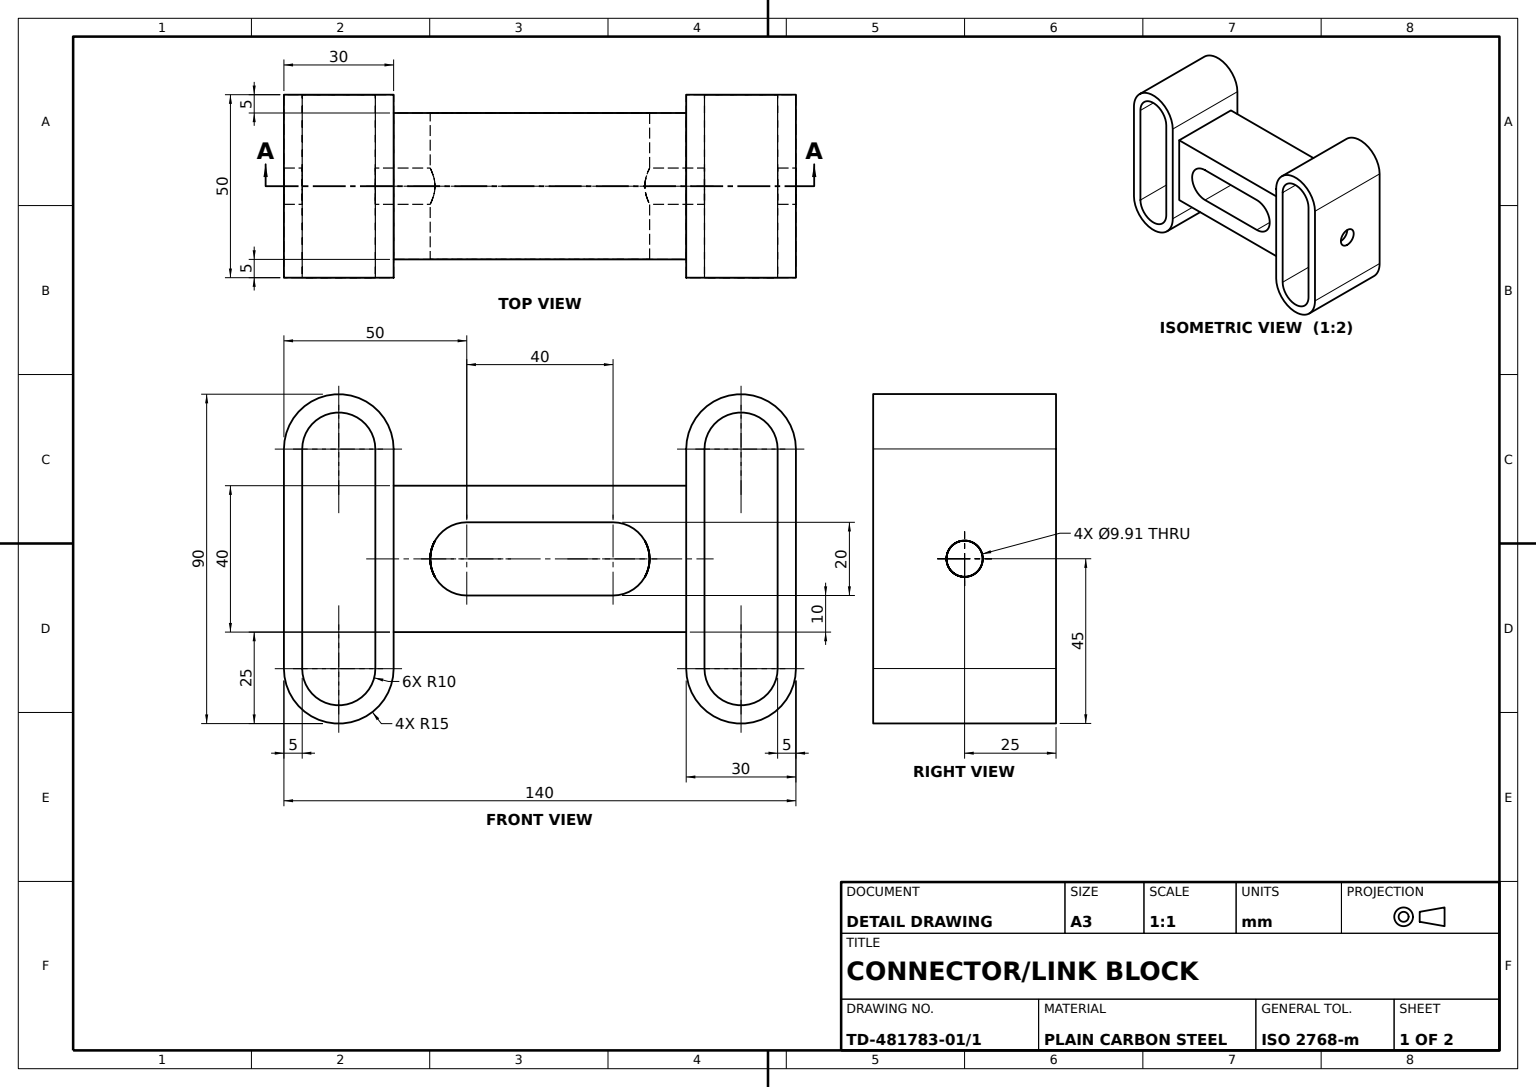
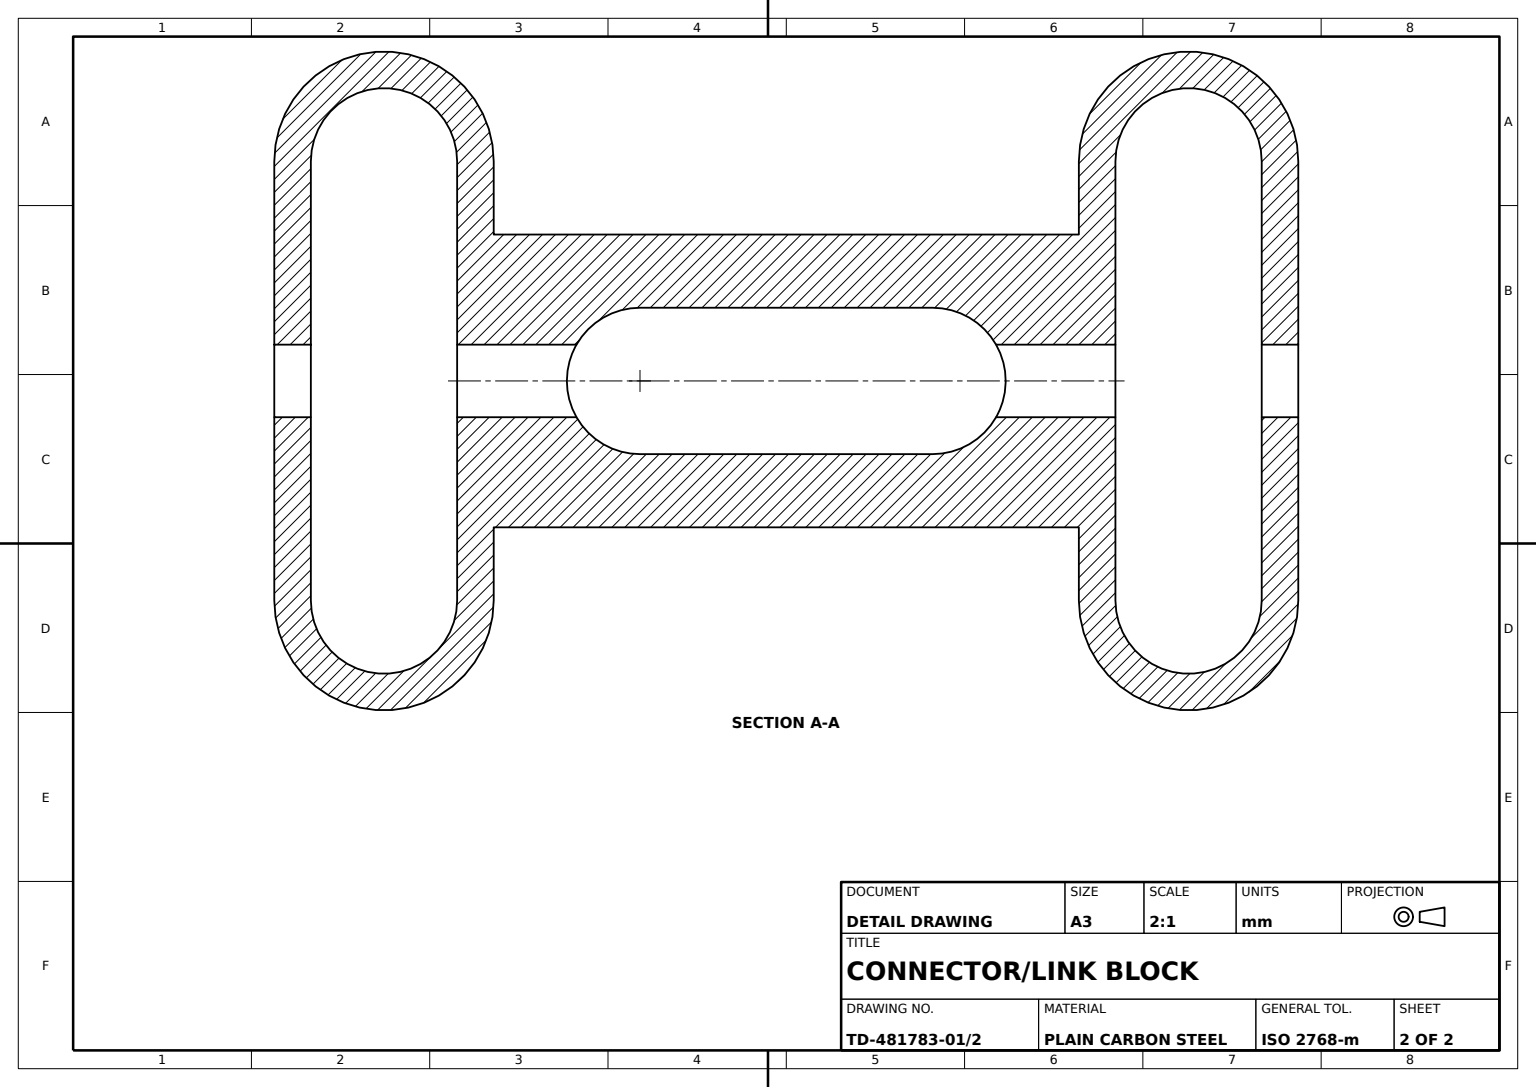
ISO-10303-21;
HEADER;
FILE_DESCRIPTION((''),'2;1');
FILE_NAME('','',(''),(''),'','','');
FILE_SCHEMA(('AUTOMOTIVE_DESIGN'));
ENDSEC;
DATA;
#1=APPLICATION_CONTEXT('');
#2=PRODUCT_CONTEXT('',#1,'mechanical');
#3=PRODUCT('','','',(#2));
#4=PRODUCT_DEFINITION_FORMATION('','',#3);
#5=PRODUCT_DEFINITION_CONTEXT('',#1,'design');
#6=PRODUCT_DEFINITION('','',#4,#5);
#7=PRODUCT_DEFINITION_SHAPE('','',#6);
#8=(LENGTH_UNIT()NAMED_UNIT(*)SI_UNIT(.MILLI.,.METRE.));
#9=(NAMED_UNIT(*)PLANE_ANGLE_UNIT()SI_UNIT($,.RADIAN.));
#10=(NAMED_UNIT(*)SI_UNIT($,.STERADIAN.)SOLID_ANGLE_UNIT());
#11=UNCERTAINTY_MEASURE_WITH_UNIT(LENGTH_MEASURE(1.E-05),#8,'distance_accuracy_value','');
#12=(GEOMETRIC_REPRESENTATION_CONTEXT(3)GLOBAL_UNCERTAINTY_ASSIGNED_CONTEXT((#11))GLOBAL_UNIT_ASSIGNED_CONTEXT((#8,#9,#10))REPRESENTATION_CONTEXT('',''));
#13=CARTESIAN_POINT('',(20.,-5.,20.));
#14=VERTEX_POINT('',#13);
#15=CARTESIAN_POINT('',(20.,15.,20.));
#16=VERTEX_POINT('',#15);
#17=CARTESIAN_POINT('',(20.,5.,20.));
#18=DIRECTION('',(0.,0.,1.));
#19=DIRECTION('',(1.,0.,0.));
#20=AXIS2_PLACEMENT_3D('',#17,#18,#19);
#21=CIRCLE('',#20,10.);
#22=EDGE_CURVE('',#14,#16,#21,.T.);
#23=ORIENTED_EDGE('',*,*,#22,.T.);
#24=CARTESIAN_POINT('',(20.,15.,-20.));
#25=VERTEX_POINT('',#24);
#26=DIRECTION('',(0.,0.,-1.));
#27=VECTOR('',#26,1000.);
#28=LINE('',#15,#27);
#29=EDGE_CURVE('',#16,#25,#28,.T.);
#30=ORIENTED_EDGE('',*,*,#29,.T.);
#31=CARTESIAN_POINT('',(20.,-5.,-20.));
#32=VERTEX_POINT('',#31);
#33=CARTESIAN_POINT('',(20.,5.,-20.));
#34=AXIS2_PLACEMENT_3D('',#33,#18,#19);
#35=CIRCLE('',#34,10.);
#36=EDGE_CURVE('',#32,#25,#35,.T.);
#37=ORIENTED_EDGE('',*,*,#36,.F.);
#38=LINE('',#13,#27);
#39=EDGE_CURVE('',#14,#32,#38,.T.);
#40=ORIENTED_EDGE('',*,*,#39,.F.);
#41=EDGE_LOOP('',(#23,#30,#37,#40));
#42=FACE_OUTER_BOUND('',#41,.T.);
#43=CARTESIAN_POINT('',(28.684746,9.957337,0.));
#44=VERTEX_POINT('',#43);
#45=CARTESIAN_POINT('',(28.684746,0.042663,0.));
#46=VERTEX_POINT('',#45);
#47=CARTESIAN_POINT('',(28.684746,9.957337,-0.333644));
#48=CARTESIAN_POINT('',(28.703997,9.924013,-0.66037));
#49=CARTESIAN_POINT('',(28.77589,9.794709,-1.30106));
#50=CARTESIAN_POINT('',(28.829393,9.69698,-1.618118));
#51=CARTESIAN_POINT('',(28.958027,9.446746,-2.215033));
#52=CARTESIAN_POINT('',(29.033067,9.294469,-2.497257));
#53=CARTESIAN_POINT('',(29.195117,8.935554,-3.03153));
#54=CARTESIAN_POINT('',(29.280861,8.73138,-3.279188));
#55=CARTESIAN_POINT('',(29.449156,8.281924,-3.728974));
#56=CARTESIAN_POINT('',(29.532956,8.033174,-3.934313));
#57=CARTESIAN_POINT('',(29.686841,7.4985,-4.29377));
#58=CARTESIAN_POINT('',(29.756046,7.216232,-4.446107));
#59=CARTESIAN_POINT('',(29.872495,6.62048,-4.696125));
#60=CARTESIAN_POINT('',(29.920076,6.302511,-4.794404));
#61=CARTESIAN_POINT('',(29.983476,5.659278,-4.924246));
#62=CARTESIAN_POINT('',(29.999894,5.333422,-4.957123));
#63=CARTESIAN_POINT('',(30.000052,4.838099,-4.957443));
#64=CARTESIAN_POINT('',(29.995941,4.670826,-4.949166));
#65=CARTESIAN_POINT('',(29.97965,4.341378,-4.916179));
#66=CARTESIAN_POINT('',(29.96753,4.17881,-4.89159));
#67=CARTESIAN_POINT('',(29.920034,3.697322,-4.794316));
#68=CARTESIAN_POINT('',(29.873005,3.382012,-4.697227));
#69=CARTESIAN_POINT('',(29.755256,2.779842,-4.444403));
#70=CARTESIAN_POINT('',(29.685595,2.496769,-4.290954));
#71=CARTESIAN_POINT('',(29.531954,1.963757,-3.93188));
#72=CARTESIAN_POINT('',(29.447628,1.713675,-3.725129));
#73=CARTESIAN_POINT('',(29.279098,1.264235,-3.274229));
#74=CARTESIAN_POINT('',(29.194094,1.06205,-3.028479));
#75=CARTESIAN_POINT('',(29.031848,0.702962,-2.49291));
#76=CARTESIAN_POINT('',(28.9566,0.550419,-2.209035));
#77=CARTESIAN_POINT('',(28.860899,0.364341,-1.764004));
#78=CARTESIAN_POINT('',(28.831773,0.309293,-1.612131));
#79=CARTESIAN_POINT('',(28.780291,0.213619,-1.30087));
#80=CARTESIAN_POINT('',(28.757825,0.172797,-1.140426));
#81=CARTESIAN_POINT('',(28.70345,0.075011,-0.654786));
#82=CARTESIAN_POINT('',(28.684746,0.042663,-0.328607));
#83=B_SPLINE_CURVE_WITH_KNOTS('',3,(#43,#47,#48,#49,#50,#51,#52,#53,#54,#55,#56,#57,#58,#59,#60,#61,#62,#63,#64,#65,#66,#67,#68,#69,#70,#71,#72,#73,#74,#75,#76,#77,#78,#79,#80,#81,#82,#45),.UNSPECIFIED.,.F.,.F.,(4,2,2,2,2,2,2,2,2,2,2,2,2,2,2,2,2,2,4),(0.,0.000985138,0.001970276,0.002955414,0.003940552,0.00492569,0.005910828,0.006895966,0.007881104,0.008373673,0.008866241,0.009851379,0.010836517,0.011821655,0.012806793,0.013791931,0.0142845,0.014777069,0.015762207),.UNSPECIFIED.);
#84=EDGE_CURVE('',#44,#46,#83,.T.);
#85=ORIENTED_EDGE('',*,*,#84,.F.);
#86=CARTESIAN_POINT('',(28.684746,0.042663,0.328046));
#87=CARTESIAN_POINT('',(28.704119,0.076197,0.662291));
#88=CARTESIAN_POINT('',(28.776349,0.206127,1.304318));
#89=CARTESIAN_POINT('',(28.828745,0.301769,1.615031));
#90=CARTESIAN_POINT('',(28.958438,0.554046,2.217025));
#91=CARTESIAN_POINT('',(29.033801,0.707138,2.499716));
#92=CARTESIAN_POINT('',(29.194673,1.063479,3.030024));
#93=CARTESIAN_POINT('',(29.28113,1.269253,3.279968));
#94=CARTESIAN_POINT('',(29.449745,1.719732,3.730483));
#95=CARTESIAN_POINT('',(29.532308,1.964884,3.932729));
#96=CARTESIAN_POINT('',(29.685793,2.497554,4.291392));
#97=CARTESIAN_POINT('',(29.756426,2.785497,4.446934));
#98=CARTESIAN_POINT('',(29.872635,3.380447,4.696413));
#99=CARTESIAN_POINT('',(29.919219,3.690438,4.792638));
#100=CARTESIAN_POINT('',(29.983364,4.337968,4.924027));
#101=CARTESIAN_POINT('',(29.999866,4.667885,4.957067));
#102=CARTESIAN_POINT('',(30.000066,5.159964,4.95747));
#103=CARTESIAN_POINT('',(29.996099,5.324148,4.949484));
#104=CARTESIAN_POINT('',(29.980024,5.652841,4.916937));
#105=CARTESIAN_POINT('',(29.967804,5.818032,4.892149));
#106=CARTESIAN_POINT('',(29.920153,6.302214,4.794565));
#107=CARTESIAN_POINT('',(29.873721,6.613467,4.698717));
#108=CARTESIAN_POINT('',(29.785869,7.064023,4.510156));
#109=CARTESIAN_POINT('',(29.753378,7.212034,4.439403));
#110=CARTESIAN_POINT('',(29.684363,7.496919,4.285649));
#111=CARTESIAN_POINT('',(29.647742,7.634422,4.202456));
#112=CARTESIAN_POINT('',(29.533004,8.032861,3.934392));
#113=CARTESIAN_POINT('',(29.449352,8.281492,3.729566));
#114=CARTESIAN_POINT('',(29.279736,8.734294,3.276111));
#115=CARTESIAN_POINT('',(29.194905,8.93597,3.030695));
#116=CARTESIAN_POINT('',(29.034217,9.291977,2.501182));
#117=CARTESIAN_POINT('',(28.957674,9.447443,2.21351));
#118=CARTESIAN_POINT('',(28.829418,9.696919,1.618124));
#119=CARTESIAN_POINT('',(28.777113,9.79248,1.309391));
#120=CARTESIAN_POINT('',(28.704547,9.923052,0.667776));
#121=CARTESIAN_POINT('',(28.684746,9.957337,0.333074));
#122=B_SPLINE_CURVE_WITH_KNOTS('',3,(#45,#86,#87,#88,#89,#90,#91,#92,#93,#94,#95,#96,#97,#98,#99,#100,#101,#102,#103,#104,#105,#106,#107,#108,#109,#110,#111,#112,#113,#114,#115,#116,#117,#118,#119,#120,#121,#43),.UNSPECIFIED.,.F.,.F.,(4,2,2,2,2,2,2,2,2,2,2,2,2,2,2,2,2,2,4),(0.015762207,0.016745662,0.017729117,0.018712571,0.019696026,0.020679481,0.021662936,0.02264639,0.023629845,0.024121573,0.0246133,0.025596755,0.026088482,0.026580209,0.027563664,0.028547119,0.029530574,0.030514029,0.031497483),.UNSPECIFIED.);
#123=EDGE_CURVE('',#46,#44,#122,.T.);
#124=ORIENTED_EDGE('',*,*,#123,.F.);
#125=EDGE_LOOP('',(#85,#124));
#126=FACE_BOUND('',#125,.T.);
#127=DIRECTION('',(-1.,0.,0.));
#128=AXIS2_PLACEMENT_3D('',#17,#26,#127);
#129=CYLINDRICAL_SURFACE('',#128,10.);
#130=ADVANCED_FACE('',(#42,#126),#129,.F.);
#131=ORIENTED_EDGE('',*,*,#29,.F.);
#132=CARTESIAN_POINT('',(-20.,15.,20.));
#133=VERTEX_POINT('',#132);
#134=VECTOR('',#127,1000.);
#135=LINE('',#132,#134);
#136=EDGE_CURVE('',#16,#133,#135,.T.);
#137=ORIENTED_EDGE('',*,*,#136,.T.);
#138=CARTESIAN_POINT('',(-20.,15.,-20.));
#139=VERTEX_POINT('',#138);
#140=LINE('',#132,#27);
#141=EDGE_CURVE('',#133,#139,#140,.T.);
#142=ORIENTED_EDGE('',*,*,#141,.T.);
#143=LINE('',#138,#134);
#144=EDGE_CURVE('',#25,#139,#143,.T.);
#145=ORIENTED_EDGE('',*,*,#144,.F.);
#146=EDGE_LOOP('',(#131,#137,#142,#145));
#147=FACE_OUTER_BOUND('',#146,.T.);
#148=DIRECTION('',(0.,-1.,0.));
#149=AXIS2_PLACEMENT_3D('',#132,#148,#19);
#150=PLANE('',#149);
#151=ADVANCED_FACE('',(#147),#150,.T.);
#152=CARTESIAN_POINT('',(65.,35.,-25.));
#153=VERTEX_POINT('',#152);
#154=CARTESIAN_POINT('',(45.,35.,-25.));
#155=VERTEX_POINT('',#154);
#156=CARTESIAN_POINT('',(55.,35.,-25.));
#157=AXIS2_PLACEMENT_3D('',#156,#18,#19);
#158=CIRCLE('',#157,10.);
#159=EDGE_CURVE('',#153,#155,#158,.T.);
#160=ORIENTED_EDGE('',*,*,#159,.F.);
#161=CARTESIAN_POINT('',(65.,35.,25.));
#162=VERTEX_POINT('',#161);
#163=LINE('',#161,#27);
#164=EDGE_CURVE('',#162,#153,#163,.T.);
#165=ORIENTED_EDGE('',*,*,#164,.F.);
#166=CARTESIAN_POINT('',(45.,35.,25.));
#167=VERTEX_POINT('',#166);
#168=CARTESIAN_POINT('',(55.,35.,25.));
#169=AXIS2_PLACEMENT_3D('',#168,#18,#19);
#170=CIRCLE('',#169,10.);
#171=EDGE_CURVE('',#162,#167,#170,.T.);
#172=ORIENTED_EDGE('',*,*,#171,.T.);
#173=LINE('',#166,#27);
#174=EDGE_CURVE('',#167,#155,#173,.T.);
#175=ORIENTED_EDGE('',*,*,#174,.T.);
#176=EDGE_LOOP('',(#160,#165,#172,#175));
#177=FACE_OUTER_BOUND('',#176,.T.);
#178=AXIS2_PLACEMENT_3D('',#168,#26,#127);
#179=CYLINDRICAL_SURFACE('',#178,10.);
#180=ADVANCED_FACE('',(#177),#179,.F.);
#181=CARTESIAN_POINT('',(-70.,0.042663,0.));
#182=VERTEX_POINT('',#181);
#183=CARTESIAN_POINT('',(-70.,9.957337,0.));
#184=VERTEX_POINT('',#183);
#185=CARTESIAN_POINT('',(-70.,5.,0.));
#186=DIRECTION('',(0.,1.,0.));
#187=AXIS2_PLACEMENT_3D('',#185,#19,#186);
#188=CIRCLE('',#187,4.957337);
#189=EDGE_CURVE('',#182,#184,#188,.T.);
#190=ORIENTED_EDGE('',*,*,#189,.F.);
#191=CARTESIAN_POINT('',(-65.,0.042663,0.));
#192=VERTEX_POINT('',#191);
#193=CARTESIAN_POINT('',(-94.,0.042663,0.));
#194=VECTOR('',#19,1000.);
#195=LINE('',#193,#194);
#196=EDGE_CURVE('',#182,#192,#195,.T.);
#197=ORIENTED_EDGE('',*,*,#196,.T.);
#198=CARTESIAN_POINT('',(-65.,9.957337,0.));
#199=VERTEX_POINT('',#198);
#200=CARTESIAN_POINT('',(-65.,5.,0.));
#201=AXIS2_PLACEMENT_3D('',#200,#19,#186);
#202=CIRCLE('',#201,4.957337);
#203=EDGE_CURVE('',#192,#199,#202,.T.);
#204=ORIENTED_EDGE('',*,*,#203,.T.);
#205=CARTESIAN_POINT('',(-94.,9.957337,0.));
#206=LINE('',#205,#194);
#207=EDGE_CURVE('',#184,#199,#206,.T.);
#208=ORIENTED_EDGE('',*,*,#207,.F.);
#209=EDGE_LOOP('',(#190,#197,#204,#208));
#210=FACE_OUTER_BOUND('',#209,.T.);
#211=CARTESIAN_POINT('',(-94.,5.,0.));
#212=AXIS2_PLACEMENT_3D('',#211,#19,#186);
#213=CYLINDRICAL_SURFACE('',#212,4.957337);
#214=ADVANCED_FACE('',(#210),#213,.F.);
#215=CARTESIAN_POINT('',(-20.,-5.,-20.));
#216=VERTEX_POINT('',#215);
#217=LINE('',#215,#194);
#218=EDGE_CURVE('',#216,#32,#217,.T.);
#219=ORIENTED_EDGE('',*,*,#218,.F.);
#220=CARTESIAN_POINT('',(-20.,-5.,20.));
#221=VERTEX_POINT('',#220);
#222=LINE('',#220,#27);
#223=EDGE_CURVE('',#221,#216,#222,.T.);
#224=ORIENTED_EDGE('',*,*,#223,.F.);
#225=LINE('',#220,#194);
#226=EDGE_CURVE('',#221,#14,#225,.T.);
#227=ORIENTED_EDGE('',*,*,#226,.T.);
#228=ORIENTED_EDGE('',*,*,#39,.T.);
#229=EDGE_LOOP('',(#219,#224,#227,#228));
#230=FACE_OUTER_BOUND('',#229,.T.);
#231=AXIS2_PLACEMENT_3D('',#220,#186,#127);
#232=PLANE('',#231);
#233=ADVANCED_FACE('',(#230),#232,.T.);
#234=CARTESIAN_POINT('',(-28.684746,9.957337,0.));
#235=VERTEX_POINT('',#234);
#236=CARTESIAN_POINT('',(-30.,5.,4.957337));
#237=VERTEX_POINT('',#236);
#238=CARTESIAN_POINT('',(-28.684746,9.957337,0.333779));
#239=CARTESIAN_POINT('',(-28.704013,9.923986,0.660635));
#240=CARTESIAN_POINT('',(-28.775961,9.794579,1.301574));
#241=CARTESIAN_POINT('',(-28.829505,9.696771,1.618748));
#242=CARTESIAN_POINT('',(-28.958226,9.446347,2.215852));
#243=CARTESIAN_POINT('',(-29.033315,9.293955,2.498158));
#244=CARTESIAN_POINT('',(-29.19546,8.934761,3.032574));
#245=CARTESIAN_POINT('',(-29.281239,8.730451,3.280258));
#246=CARTESIAN_POINT('',(-29.449596,8.280671,3.730087));
#247=CARTESIAN_POINT('',(-29.533423,8.031721,3.935443));
#248=CARTESIAN_POINT('',(-29.687308,7.496708,4.294821));
#249=CARTESIAN_POINT('',(-29.7565,7.214259,4.4471));
#250=CARTESIAN_POINT('',(-29.872889,6.618113,4.696952));
#251=CARTESIAN_POINT('',(-29.920419,6.299933,4.795112));
#252=CARTESIAN_POINT('',(-29.983671,5.656391,4.924639));
#253=CARTESIAN_POINT('',(-30.,5.330377,4.957337));
#254=B_SPLINE_CURVE_WITH_KNOTS('',3,(#234,#238,#239,#240,#241,#242,#243,#244,#245,#246,#247,#248,#249,#250,#251,#252,#253,#236),.UNSPECIFIED.,.F.,.F.,(4,2,2,2,2,2,2,2,4),(0.,0.000985537,0.001971073,0.00295661,0.003942146,0.004927683,0.005913219,0.006898756,0.007884292),.UNSPECIFIED.);
#255=EDGE_CURVE('',#235,#237,#254,.T.);
#256=ORIENTED_EDGE('',*,*,#255,.F.);
#257=CARTESIAN_POINT('',(-30.,5.,-4.957337));
#258=VERTEX_POINT('',#257);
#259=CARTESIAN_POINT('',(-30.,5.163944,-4.957337));
#260=CARTESIAN_POINT('',(-29.995971,5.328047,-4.949225));
#261=CARTESIAN_POINT('',(-29.979777,5.656575,-4.916437));
#262=CARTESIAN_POINT('',(-29.967504,5.821655,-4.891538));
#263=CARTESIAN_POINT('',(-29.919719,6.305461,-4.793668));
#264=CARTESIAN_POINT('',(-29.873222,6.61648,-4.69767));
#265=CARTESIAN_POINT('',(-29.785302,7.066701,-4.508927));
#266=CARTESIAN_POINT('',(-29.752797,7.214588,-4.438125));
#267=CARTESIAN_POINT('',(-29.683769,7.499214,-4.284307));
#268=CARTESIAN_POINT('',(-29.647147,7.636595,-4.20109));
#269=CARTESIAN_POINT('',(-29.532418,8.034683,-3.932973));
#270=CARTESIAN_POINT('',(-29.448783,8.283114,-3.728123));
#271=CARTESIAN_POINT('',(-29.279255,8.735475,-3.274746));
#272=CARTESIAN_POINT('',(-29.194476,8.936963,-3.029389));
#273=CARTESIAN_POINT('',(-29.033899,9.292637,-2.500028));
#274=CARTESIAN_POINT('',(-28.957418,9.447954,-2.212457));
#275=CARTESIAN_POINT('',(-28.829277,9.69718,-1.617333));
#276=CARTESIAN_POINT('',(-28.777021,9.792647,-1.308741));
#277=CARTESIAN_POINT('',(-28.704526,9.923088,-0.667433));
#278=CARTESIAN_POINT('',(-28.684746,9.957337,-0.332902));
#279=B_SPLINE_CURVE_WITH_KNOTS('',3,(#257,#259,#260,#261,#262,#263,#264,#265,#266,#267,#268,#269,#270,#271,#272,#273,#274,#275,#276,#277,#278,#234),.UNSPECIFIED.,.F.,.F.,(4,2,2,2,2,2,2,2,2,2,4),(0.023633905,0.024125379,0.024616852,0.0255998,0.026091273,0.026582747,0.027565694,0.028548641,0.029531589,0.030514536,0.031497483),.UNSPECIFIED.);
#280=EDGE_CURVE('',#258,#235,#279,.T.);
#281=ORIENTED_EDGE('',*,*,#280,.F.);
#282=CARTESIAN_POINT('',(-30.,5.,-20.));
#283=VERTEX_POINT('',#282);
#284=CARTESIAN_POINT('',(-30.,5.,20.));
#285=LINE('',#284,#27);
#286=EDGE_CURVE('',#258,#283,#285,.T.);
#287=ORIENTED_EDGE('',*,*,#286,.T.);
#288=CARTESIAN_POINT('',(-20.,5.,-20.));
#289=AXIS2_PLACEMENT_3D('',#288,#18,#19);
#290=CIRCLE('',#289,10.);
#291=EDGE_CURVE('',#139,#283,#290,.T.);
#292=ORIENTED_EDGE('',*,*,#291,.F.);
#293=ORIENTED_EDGE('',*,*,#141,.F.);
#294=VERTEX_POINT('',#284);
#295=CARTESIAN_POINT('',(-20.,5.,20.));
#296=AXIS2_PLACEMENT_3D('',#295,#18,#19);
#297=CIRCLE('',#296,10.);
#298=EDGE_CURVE('',#133,#294,#297,.T.);
#299=ORIENTED_EDGE('',*,*,#298,.T.);
#300=EDGE_CURVE('',#294,#237,#285,.T.);
#301=ORIENTED_EDGE('',*,*,#300,.T.);
#302=EDGE_LOOP('',(#256,#281,#287,#292,#293,#299,#301));
#303=FACE_OUTER_BOUND('',#302,.T.);
#304=AXIS2_PLACEMENT_3D('',#295,#26,#127);
#305=CYLINDRICAL_SURFACE('',#304,10.);
#306=ADVANCED_FACE('',(#303),#305,.F.);
#307=CARTESIAN_POINT('',(-40.,35.,25.));
#308=VERTEX_POINT('',#307);
#309=CARTESIAN_POINT('',(-70.,35.,25.));
#310=VERTEX_POINT('',#309);
#311=CARTESIAN_POINT('',(-55.,35.,25.));
#312=AXIS2_PLACEMENT_3D('',#311,#18,#19);
#313=CIRCLE('',#312,15.);
#314=EDGE_CURVE('',#308,#310,#313,.T.);
#315=ORIENTED_EDGE('',*,*,#314,.F.);
#316=CARTESIAN_POINT('',(-40.,35.,-25.));
#317=VERTEX_POINT('',#316);
#318=LINE('',#307,#27);
#319=EDGE_CURVE('',#308,#317,#318,.T.);
#320=ORIENTED_EDGE('',*,*,#319,.T.);
#321=CARTESIAN_POINT('',(-70.,35.,-25.));
#322=VERTEX_POINT('',#321);
#323=CARTESIAN_POINT('',(-55.,35.,-25.));
#324=AXIS2_PLACEMENT_3D('',#323,#18,#19);
#325=CIRCLE('',#324,15.);
#326=EDGE_CURVE('',#317,#322,#325,.T.);
#327=ORIENTED_EDGE('',*,*,#326,.T.);
#328=LINE('',#309,#27);
#329=EDGE_CURVE('',#310,#322,#328,.T.);
#330=ORIENTED_EDGE('',*,*,#329,.F.);
#331=EDGE_LOOP('',(#315,#320,#327,#330));
#332=FACE_OUTER_BOUND('',#331,.T.);
#333=AXIS2_PLACEMENT_3D('',#311,#26,#127);
#334=CYLINDRICAL_SURFACE('',#333,15.);
#335=ADVANCED_FACE('',(#332),#334,.T.);
#336=CARTESIAN_POINT('',(40.,-25.,25.));
#337=VERTEX_POINT('',#336);
#338=CARTESIAN_POINT('',(40.,-25.,-25.));
#339=VERTEX_POINT('',#338);
#340=LINE('',#336,#27);
#341=EDGE_CURVE('',#337,#339,#340,.T.);
#342=ORIENTED_EDGE('',*,*,#341,.F.);
#343=CARTESIAN_POINT('',(40.,35.,25.));
#344=VERTEX_POINT('',#343);
#345=CARTESIAN_POINT('',(40.,0.,25.));
#346=VECTOR('',#148,1000.);
#347=LINE('',#345,#346);
#348=EDGE_CURVE('',#344,#337,#347,.T.);
#349=ORIENTED_EDGE('',*,*,#348,.F.);
#350=CARTESIAN_POINT('',(40.,35.,-25.));
#351=VERTEX_POINT('',#350);
#352=LINE('',#343,#27);
#353=EDGE_CURVE('',#344,#351,#352,.T.);
#354=ORIENTED_EDGE('',*,*,#353,.T.);
#355=CARTESIAN_POINT('',(40.,0.,-25.));
#356=LINE('',#355,#346);
#357=EDGE_CURVE('',#351,#339,#356,.T.);
#358=ORIENTED_EDGE('',*,*,#357,.T.);
#359=EDGE_LOOP('',(#342,#349,#354,#358));
#360=FACE_OUTER_BOUND('',#359,.T.);
#361=CARTESIAN_POINT('',(40.,-15.,-20.));
#362=VERTEX_POINT('',#361);
#363=CARTESIAN_POINT('',(40.,25.,-20.));
#364=VERTEX_POINT('',#363);
#365=VECTOR('',#186,1000.);
#366=LINE('',#363,#365);
#367=EDGE_CURVE('',#362,#364,#366,.T.);
#368=ORIENTED_EDGE('',*,*,#367,.T.);
#369=CARTESIAN_POINT('',(40.,25.,20.));
#370=VERTEX_POINT('',#369);
#371=LINE('',#369,#27);
#372=EDGE_CURVE('',#370,#364,#371,.T.);
#373=ORIENTED_EDGE('',*,*,#372,.F.);
#374=CARTESIAN_POINT('',(40.,-15.,20.));
#375=VERTEX_POINT('',#374);
#376=LINE('',#369,#365);
#377=EDGE_CURVE('',#375,#370,#376,.T.);
#378=ORIENTED_EDGE('',*,*,#377,.F.);
#379=LINE('',#374,#27);
#380=EDGE_CURVE('',#375,#362,#379,.T.);
#381=ORIENTED_EDGE('',*,*,#380,.T.);
#382=EDGE_LOOP('',(#368,#373,#378,#381));
#383=FACE_BOUND('',#382,.T.);
#384=AXIS2_PLACEMENT_3D('',#345,#19,#186);
#385=PLANE('',#384);
#386=ADVANCED_FACE('',(#360,#383),#385,.F.);
#387=CARTESIAN_POINT('',(-45.,0.042663,0.));
#388=VERTEX_POINT('',#387);
#389=CARTESIAN_POINT('',(-45.,9.957337,0.));
#390=VERTEX_POINT('',#389);
#391=CARTESIAN_POINT('',(-45.,5.,0.));
#392=AXIS2_PLACEMENT_3D('',#391,#19,#186);
#393=CIRCLE('',#392,4.957337);
#394=EDGE_CURVE('',#388,#390,#393,.T.);
#395=ORIENTED_EDGE('',*,*,#394,.T.);
#396=EDGE_CURVE('',#390,#388,#393,.T.);
#397=ORIENTED_EDGE('',*,*,#396,.T.);
#398=EDGE_LOOP('',(#395,#397));
#399=FACE_BOUND('',#398,.T.);
#400=CARTESIAN_POINT('',(-45.,35.,-25.));
#401=VERTEX_POINT('',#400);
#402=CARTESIAN_POINT('',(-45.,-25.,-25.));
#403=VERTEX_POINT('',#402);
#404=CARTESIAN_POINT('',(-45.,0.,-25.));
#405=LINE('',#404,#346);
#406=EDGE_CURVE('',#401,#403,#405,.T.);
#407=ORIENTED_EDGE('',*,*,#406,.T.);
#408=CARTESIAN_POINT('',(-45.,-25.,25.));
#409=VERTEX_POINT('',#408);
#410=LINE('',#408,#27);
#411=EDGE_CURVE('',#409,#403,#410,.T.);
#412=ORIENTED_EDGE('',*,*,#411,.F.);
#413=CARTESIAN_POINT('',(-45.,35.,25.));
#414=VERTEX_POINT('',#413);
#415=CARTESIAN_POINT('',(-45.,0.,25.));
#416=LINE('',#415,#346);
#417=EDGE_CURVE('',#414,#409,#416,.T.);
#418=ORIENTED_EDGE('',*,*,#417,.F.);
#419=LINE('',#413,#27);
#420=EDGE_CURVE('',#414,#401,#419,.T.);
#421=ORIENTED_EDGE('',*,*,#420,.T.);
#422=EDGE_LOOP('',(#407,#412,#418,#421));
#423=FACE_OUTER_BOUND('',#422,.T.);
#424=AXIS2_PLACEMENT_3D('',#415,#19,#186);
#425=PLANE('',#424);
#426=ADVANCED_FACE('',(#399,#423),#425,.F.);
#427=ORIENTED_EDGE('',*,*,#189,.T.);
#428=EDGE_CURVE('',#184,#182,#188,.T.);
#429=ORIENTED_EDGE('',*,*,#428,.T.);
#430=EDGE_LOOP('',(#427,#429));
#431=FACE_BOUND('',#430,.T.);
#432=CARTESIAN_POINT('',(-70.,-25.,-25.));
#433=VERTEX_POINT('',#432);
#434=CARTESIAN_POINT('',(-70.,0.,-25.));
#435=LINE('',#434,#346);
#436=EDGE_CURVE('',#322,#433,#435,.T.);
#437=ORIENTED_EDGE('',*,*,#436,.T.);
#438=CARTESIAN_POINT('',(-70.,-25.,25.));
#439=VERTEX_POINT('',#438);
#440=LINE('',#438,#27);
#441=EDGE_CURVE('',#439,#433,#440,.T.);
#442=ORIENTED_EDGE('',*,*,#441,.F.);
#443=CARTESIAN_POINT('',(-70.,0.,25.));
#444=LINE('',#443,#346);
#445=EDGE_CURVE('',#310,#439,#444,.T.);
#446=ORIENTED_EDGE('',*,*,#445,.F.);
#447=ORIENTED_EDGE('',*,*,#329,.T.);
#448=EDGE_LOOP('',(#437,#442,#446,#447));
#449=FACE_OUTER_BOUND('',#448,.T.);
#450=AXIS2_PLACEMENT_3D('',#443,#19,#186);
#451=PLANE('',#450);
#452=ADVANCED_FACE('',(#431,#449),#451,.F.);
#453=CARTESIAN_POINT('',(70.,35.,-25.));
#454=VERTEX_POINT('',#453);
#455=CIRCLE('',#157,15.);
#456=EDGE_CURVE('',#454,#351,#455,.T.);
#457=ORIENTED_EDGE('',*,*,#456,.T.);
#458=ORIENTED_EDGE('',*,*,#353,.F.);
#459=CARTESIAN_POINT('',(70.,35.,25.));
#460=VERTEX_POINT('',#459);
#461=CIRCLE('',#169,15.);
#462=EDGE_CURVE('',#460,#344,#461,.T.);
#463=ORIENTED_EDGE('',*,*,#462,.F.);
#464=LINE('',#459,#27);
#465=EDGE_CURVE('',#460,#454,#464,.T.);
#466=ORIENTED_EDGE('',*,*,#465,.T.);
#467=EDGE_LOOP('',(#457,#458,#463,#466));
#468=FACE_OUTER_BOUND('',#467,.T.);
#469=CYLINDRICAL_SURFACE('',#178,15.);
#470=ADVANCED_FACE('',(#468),#469,.T.);
#471=CARTESIAN_POINT('',(-40.,-25.,25.));
#472=VERTEX_POINT('',#471);
#473=CARTESIAN_POINT('',(-40.,-25.,-25.));
#474=VERTEX_POINT('',#473);
#475=LINE('',#471,#27);
#476=EDGE_CURVE('',#472,#474,#475,.T.);
#477=ORIENTED_EDGE('',*,*,#476,.T.);
#478=CARTESIAN_POINT('',(-40.,0.,-25.));
#479=LINE('',#478,#346);
#480=EDGE_CURVE('',#317,#474,#479,.T.);
#481=ORIENTED_EDGE('',*,*,#480,.F.);
#482=ORIENTED_EDGE('',*,*,#319,.F.);
#483=CARTESIAN_POINT('',(-40.,0.,25.));
#484=LINE('',#483,#346);
#485=EDGE_CURVE('',#308,#472,#484,.T.);
#486=ORIENTED_EDGE('',*,*,#485,.T.);
#487=EDGE_LOOP('',(#477,#481,#482,#486));
#488=FACE_OUTER_BOUND('',#487,.T.);
#489=CARTESIAN_POINT('',(-40.,25.,20.));
#490=VERTEX_POINT('',#489);
#491=CARTESIAN_POINT('',(-40.,25.,-20.));
#492=VERTEX_POINT('',#491);
#493=LINE('',#489,#27);
#494=EDGE_CURVE('',#490,#492,#493,.T.);
#495=ORIENTED_EDGE('',*,*,#494,.T.);
#496=CARTESIAN_POINT('',(-40.,-15.,-20.));
#497=VERTEX_POINT('',#496);
#498=LINE('',#491,#346);
#499=EDGE_CURVE('',#492,#497,#498,.T.);
#500=ORIENTED_EDGE('',*,*,#499,.T.);
#501=CARTESIAN_POINT('',(-40.,-15.,20.));
#502=VERTEX_POINT('',#501);
#503=LINE('',#501,#27);
#504=EDGE_CURVE('',#502,#497,#503,.T.);
#505=ORIENTED_EDGE('',*,*,#504,.F.);
#506=LINE('',#489,#346);
#507=EDGE_CURVE('',#490,#502,#506,.T.);
#508=ORIENTED_EDGE('',*,*,#507,.F.);
#509=EDGE_LOOP('',(#495,#500,#505,#508));
#510=FACE_BOUND('',#509,.T.);
#511=AXIS2_PLACEMENT_3D('',#483,#19,#186);
#512=PLANE('',#511);
#513=ADVANCED_FACE('',(#488,#510),#512,.T.);
#514=CARTESIAN_POINT('',(70.,-25.,25.));
#515=VERTEX_POINT('',#514);
#516=CARTESIAN_POINT('',(55.,-25.,25.));
#517=AXIS2_PLACEMENT_3D('',#516,#18,#19);
#518=CIRCLE('',#517,15.);
#519=EDGE_CURVE('',#337,#515,#518,.T.);
#520=ORIENTED_EDGE('',*,*,#519,.T.);
#521=CARTESIAN_POINT('',(70.,0.,25.));
#522=LINE('',#521,#346);
#523=EDGE_CURVE('',#460,#515,#522,.T.);
#524=ORIENTED_EDGE('',*,*,#523,.F.);
#525=ORIENTED_EDGE('',*,*,#462,.T.);
#526=ORIENTED_EDGE('',*,*,#348,.T.);
#527=EDGE_LOOP('',(#520,#524,#525,#526));
#528=FACE_OUTER_BOUND('',#527,.T.);
#529=ORIENTED_EDGE('',*,*,#171,.F.);
#530=CARTESIAN_POINT('',(65.,-25.,25.));
#531=VERTEX_POINT('',#530);
#532=CARTESIAN_POINT('',(65.,0.,25.));
#533=LINE('',#532,#346);
#534=EDGE_CURVE('',#162,#531,#533,.T.);
#535=ORIENTED_EDGE('',*,*,#534,.T.);
#536=CARTESIAN_POINT('',(45.,-25.,25.));
#537=VERTEX_POINT('',#536);
#538=CIRCLE('',#517,10.);
#539=EDGE_CURVE('',#537,#531,#538,.T.);
#540=ORIENTED_EDGE('',*,*,#539,.F.);
#541=CARTESIAN_POINT('',(45.,0.,25.));
#542=LINE('',#541,#346);
#543=EDGE_CURVE('',#167,#537,#542,.T.);
#544=ORIENTED_EDGE('',*,*,#543,.F.);
#545=EDGE_LOOP('',(#529,#535,#540,#544));
#546=FACE_BOUND('',#545,.T.);
#547=CARTESIAN_POINT('',(0.,0.,25.));
#548=AXIS2_PLACEMENT_3D('',#547,#18,#19);
#549=PLANE('',#548);
#550=ADVANCED_FACE('',(#528,#546),#549,.T.);
#551=CARTESIAN_POINT('',(45.,-25.,-25.));
#552=VERTEX_POINT('',#551);
#553=CARTESIAN_POINT('',(45.,0.,-25.));
#554=LINE('',#553,#346);
#555=EDGE_CURVE('',#155,#552,#554,.T.);
#556=ORIENTED_EDGE('',*,*,#555,.T.);
#557=CARTESIAN_POINT('',(65.,-25.,-25.));
#558=VERTEX_POINT('',#557);
#559=CARTESIAN_POINT('',(55.,-25.,-25.));
#560=AXIS2_PLACEMENT_3D('',#559,#18,#19);
#561=CIRCLE('',#560,10.);
#562=EDGE_CURVE('',#552,#558,#561,.T.);
#563=ORIENTED_EDGE('',*,*,#562,.T.);
#564=CARTESIAN_POINT('',(65.,0.,-25.));
#565=LINE('',#564,#346);
#566=EDGE_CURVE('',#153,#558,#565,.T.);
#567=ORIENTED_EDGE('',*,*,#566,.F.);
#568=ORIENTED_EDGE('',*,*,#159,.T.);
#569=EDGE_LOOP('',(#556,#563,#567,#568));
#570=FACE_BOUND('',#569,.T.);
#571=ORIENTED_EDGE('',*,*,#357,.F.);
#572=ORIENTED_EDGE('',*,*,#456,.F.);
#573=CARTESIAN_POINT('',(70.,-25.,-25.));
#574=VERTEX_POINT('',#573);
#575=CARTESIAN_POINT('',(70.,0.,-25.));
#576=LINE('',#575,#346);
#577=EDGE_CURVE('',#454,#574,#576,.T.);
#578=ORIENTED_EDGE('',*,*,#577,.T.);
#579=CIRCLE('',#560,15.);
#580=EDGE_CURVE('',#339,#574,#579,.T.);
#581=ORIENTED_EDGE('',*,*,#580,.F.);
#582=EDGE_LOOP('',(#571,#572,#578,#581));
#583=FACE_OUTER_BOUND('',#582,.T.);
#584=CARTESIAN_POINT('',(0.,0.,-25.));
#585=AXIS2_PLACEMENT_3D('',#584,#18,#19);
#586=PLANE('',#585);
#587=ADVANCED_FACE('',(#570,#583),#586,.F.);
#588=CARTESIAN_POINT('',(-65.,35.,25.));
#589=VERTEX_POINT('',#588);
#590=CIRCLE('',#312,10.);
#591=EDGE_CURVE('',#414,#589,#590,.T.);
#592=ORIENTED_EDGE('',*,*,#591,.T.);
#593=CARTESIAN_POINT('',(-65.,35.,-25.));
#594=VERTEX_POINT('',#593);
#595=LINE('',#588,#27);
#596=EDGE_CURVE('',#589,#594,#595,.T.);
#597=ORIENTED_EDGE('',*,*,#596,.T.);
#598=CIRCLE('',#324,10.);
#599=EDGE_CURVE('',#401,#594,#598,.T.);
#600=ORIENTED_EDGE('',*,*,#599,.F.);
#601=ORIENTED_EDGE('',*,*,#420,.F.);
#602=EDGE_LOOP('',(#592,#597,#600,#601));
#603=FACE_OUTER_BOUND('',#602,.T.);
#604=CYLINDRICAL_SURFACE('',#333,10.);
#605=ADVANCED_FACE('',(#603),#604,.F.);
#606=EDGE_CURVE('',#199,#192,#202,.T.);
#607=ORIENTED_EDGE('',*,*,#606,.F.);
#608=ORIENTED_EDGE('',*,*,#203,.F.);
#609=EDGE_LOOP('',(#607,#608));
#610=FACE_BOUND('',#609,.T.);
#611=ORIENTED_EDGE('',*,*,#596,.F.);
#612=CARTESIAN_POINT('',(-65.,-25.,25.));
#613=VERTEX_POINT('',#612);
#614=CARTESIAN_POINT('',(-65.,0.,25.));
#615=LINE('',#614,#346);
#616=EDGE_CURVE('',#589,#613,#615,.T.);
#617=ORIENTED_EDGE('',*,*,#616,.T.);
#618=CARTESIAN_POINT('',(-65.,-25.,-25.));
#619=VERTEX_POINT('',#618);
#620=LINE('',#612,#27);
#621=EDGE_CURVE('',#613,#619,#620,.T.);
#622=ORIENTED_EDGE('',*,*,#621,.T.);
#623=CARTESIAN_POINT('',(-65.,0.,-25.));
#624=LINE('',#623,#346);
#625=EDGE_CURVE('',#594,#619,#624,.T.);
#626=ORIENTED_EDGE('',*,*,#625,.F.);
#627=EDGE_LOOP('',(#611,#617,#622,#626));
#628=FACE_OUTER_BOUND('',#627,.T.);
#629=AXIS2_PLACEMENT_3D('',#614,#19,#186);
#630=PLANE('',#629);
#631=ADVANCED_FACE('',(#610,#628),#630,.T.);
#632=ORIENTED_EDGE('',*,*,#22,.F.);
#633=ORIENTED_EDGE('',*,*,#226,.F.);
#634=EDGE_CURVE('',#294,#221,#297,.T.);
#635=ORIENTED_EDGE('',*,*,#634,.F.);
#636=ORIENTED_EDGE('',*,*,#298,.F.);
#637=ORIENTED_EDGE('',*,*,#136,.F.);
#638=EDGE_LOOP('',(#632,#633,#635,#636,#637));
#639=FACE_BOUND('',#638,.T.);
#640=ORIENTED_EDGE('',*,*,#507,.T.);
#641=LINE('',#501,#194);
#642=EDGE_CURVE('',#502,#375,#641,.T.);
#643=ORIENTED_EDGE('',*,*,#642,.T.);
#644=ORIENTED_EDGE('',*,*,#377,.T.);
#645=LINE('',#489,#134);
#646=EDGE_CURVE('',#370,#490,#645,.T.);
#647=ORIENTED_EDGE('',*,*,#646,.T.);
#648=EDGE_LOOP('',(#640,#643,#644,#647));
#649=FACE_OUTER_BOUND('',#648,.T.);
#650=CARTESIAN_POINT('',(0.,0.,20.));
#651=AXIS2_PLACEMENT_3D('',#650,#18,#19);
#652=PLANE('',#651);
#653=ADVANCED_FACE('',(#639,#649),#652,.T.);
#654=CARTESIAN_POINT('',(45.,9.957337,0.));
#655=VERTEX_POINT('',#654);
#656=CARTESIAN_POINT('',(45.,0.042663,0.));
#657=VERTEX_POINT('',#656);
#658=CARTESIAN_POINT('',(45.,5.,0.));
#659=AXIS2_PLACEMENT_3D('',#658,#19,#186);
#660=CIRCLE('',#659,4.957337);
#661=EDGE_CURVE('',#655,#657,#660,.T.);
#662=ORIENTED_EDGE('',*,*,#661,.F.);
#663=EDGE_CURVE('',#657,#655,#660,.T.);
#664=ORIENTED_EDGE('',*,*,#663,.F.);
#665=EDGE_LOOP('',(#662,#664));
#666=FACE_BOUND('',#665,.T.);
#667=LINE('',#536,#27);
#668=EDGE_CURVE('',#537,#552,#667,.T.);
#669=ORIENTED_EDGE('',*,*,#668,.T.);
#670=ORIENTED_EDGE('',*,*,#555,.F.);
#671=ORIENTED_EDGE('',*,*,#174,.F.);
#672=ORIENTED_EDGE('',*,*,#543,.T.);
#673=EDGE_LOOP('',(#669,#670,#671,#672));
#674=FACE_OUTER_BOUND('',#673,.T.);
#675=AXIS2_PLACEMENT_3D('',#541,#19,#186);
#676=PLANE('',#675);
#677=ADVANCED_FACE('',(#666,#674),#676,.T.);
#678=ORIENTED_EDGE('',*,*,#280,.T.);
#679=EDGE_CURVE('',#390,#235,#206,.T.);
#680=ORIENTED_EDGE('',*,*,#679,.F.);
#681=ORIENTED_EDGE('',*,*,#394,.F.);
#682=CARTESIAN_POINT('',(-28.684746,0.042663,0.));
#683=VERTEX_POINT('',#682);
#684=EDGE_CURVE('',#388,#683,#195,.T.);
#685=ORIENTED_EDGE('',*,*,#684,.T.);
#686=CARTESIAN_POINT('',(-28.684746,0.042663,-0.328215));
#687=CARTESIAN_POINT('',(-28.70414,0.076232,-0.662633));
#688=CARTESIAN_POINT('',(-28.776441,0.206293,-1.30497));
#689=CARTESIAN_POINT('',(-28.828887,0.302031,-1.615828));
#690=CARTESIAN_POINT('',(-28.958698,0.554566,-2.218092));
#691=CARTESIAN_POINT('',(-29.034116,0.707795,-2.500864));
#692=CARTESIAN_POINT('',(-29.195105,1.064477,-3.031338));
#693=CARTESIAN_POINT('',(-29.281615,1.270449,-3.281343));
#694=CARTESIAN_POINT('',(-29.450303,1.721326,-3.731898));
#695=CARTESIAN_POINT('',(-29.532892,1.966698,-3.934144));
#696=CARTESIAN_POINT('',(-29.686396,2.499864,-4.292753));
#697=CARTESIAN_POINT('',(-29.757007,2.788028,-4.448206));
#698=CARTESIAN_POINT('',(-29.873132,3.383443,-4.697456));
#699=CARTESIAN_POINT('',(-29.919655,3.693679,-4.793538));
#700=CARTESIAN_POINT('',(-29.983623,4.341744,-4.924549));
#701=CARTESIAN_POINT('',(-30.,4.671773,-4.957337));
#702=B_SPLINE_CURVE_WITH_KNOTS('',3,(#682,#686,#687,#688,#689,#690,#691,#692,#693,#694,#695,#696,#697,#698,#699,#700,#701,#257),.UNSPECIFIED.,.F.,.F.,(4,2,2,2,2,2,2,2,4),(0.015762207,0.016746169,0.017730132,0.018714094,0.019698056,0.020682018,0.02166598,0.022649943,0.023633905),.UNSPECIFIED.);
#703=EDGE_CURVE('',#683,#258,#702,.T.);
#704=ORIENTED_EDGE('',*,*,#703,.T.);
#705=EDGE_LOOP('',(#678,#680,#681,#685,#704));
#706=FACE_OUTER_BOUND('',#705,.T.);
#707=ADVANCED_FACE('',(#706),#213,.F.);
#708=CARTESIAN_POINT('',(-55.,-25.,25.));
#709=AXIS2_PLACEMENT_3D('',#708,#18,#19);
#710=CIRCLE('',#709,15.);
#711=EDGE_CURVE('',#439,#472,#710,.T.);
#712=ORIENTED_EDGE('',*,*,#711,.F.);
#713=ORIENTED_EDGE('',*,*,#441,.T.);
#714=CARTESIAN_POINT('',(-55.,-25.,-25.));
#715=AXIS2_PLACEMENT_3D('',#714,#18,#19);
#716=CIRCLE('',#715,15.);
#717=EDGE_CURVE('',#433,#474,#716,.T.);
#718=ORIENTED_EDGE('',*,*,#717,.T.);
#719=ORIENTED_EDGE('',*,*,#476,.F.);
#720=EDGE_LOOP('',(#712,#713,#718,#719));
#721=FACE_OUTER_BOUND('',#720,.T.);
#722=AXIS2_PLACEMENT_3D('',#708,#26,#127);
#723=CYLINDRICAL_SURFACE('',#722,15.);
#724=ADVANCED_FACE('',(#721),#723,.T.);
#725=ORIENTED_EDGE('',*,*,#717,.F.);
#726=ORIENTED_EDGE('',*,*,#436,.F.);
#727=ORIENTED_EDGE('',*,*,#326,.F.);
#728=ORIENTED_EDGE('',*,*,#480,.T.);
#729=EDGE_LOOP('',(#725,#726,#727,#728));
#730=FACE_OUTER_BOUND('',#729,.T.);
#731=ORIENTED_EDGE('',*,*,#599,.T.);
#732=ORIENTED_EDGE('',*,*,#625,.T.);
#733=CIRCLE('',#715,10.);
#734=EDGE_CURVE('',#619,#403,#733,.T.);
#735=ORIENTED_EDGE('',*,*,#734,.T.);
#736=ORIENTED_EDGE('',*,*,#406,.F.);
#737=EDGE_LOOP('',(#731,#732,#735,#736));
#738=FACE_BOUND('',#737,.T.);
#739=ADVANCED_FACE('',(#730,#738),#586,.F.);
#740=ORIENTED_EDGE('',*,*,#300,.F.);
#741=ORIENTED_EDGE('',*,*,#634,.T.);
#742=ORIENTED_EDGE('',*,*,#223,.T.);
#743=EDGE_CURVE('',#283,#216,#290,.T.);
#744=ORIENTED_EDGE('',*,*,#743,.F.);
#745=ORIENTED_EDGE('',*,*,#286,.F.);
#746=ORIENTED_EDGE('',*,*,#703,.F.);
#747=CARTESIAN_POINT('',(-30.,4.834945,4.957337));
#748=CARTESIAN_POINT('',(-29.995838,4.667734,4.948956));
#749=CARTESIAN_POINT('',(-29.979456,4.338472,4.915786));
#750=CARTESIAN_POINT('',(-29.967296,4.175994,4.891114));
#751=CARTESIAN_POINT('',(-29.919693,3.694772,4.793612));
#752=CARTESIAN_POINT('',(-29.872605,3.379609,4.696387));
#753=CARTESIAN_POINT('',(-29.754798,2.77786,4.443401));
#754=CARTESIAN_POINT('',(-29.685127,2.494976,4.289898));
#755=CARTESIAN_POINT('',(-29.53149,1.962315,3.930756));
#756=CARTESIAN_POINT('',(-29.447187,1.712419,3.72401));
#757=CARTESIAN_POINT('',(-29.278721,1.263308,3.273159));
#758=CARTESIAN_POINT('',(-29.193756,1.061268,3.027449));
#759=CARTESIAN_POINT('',(-29.031595,0.702437,2.491989));
#760=CARTESIAN_POINT('',(-28.956402,0.550023,2.208217));
#761=CARTESIAN_POINT('',(-28.860766,0.364088,1.763333));
#762=CARTESIAN_POINT('',(-28.831661,0.309082,1.611511));
#763=CARTESIAN_POINT('',(-28.780216,0.213482,1.300357));
#764=CARTESIAN_POINT('',(-28.757767,0.172691,1.139968));
#765=CARTESIAN_POINT('',(-28.703435,0.074985,0.654522));
#766=CARTESIAN_POINT('',(-28.684746,0.042663,0.328474));
#767=B_SPLINE_CURVE_WITH_KNOTS('',3,(#236,#747,#748,#749,#750,#751,#752,#753,#754,#755,#756,#757,#758,#759,#760,#761,#762,#763,#764,#765,#766,#682),.UNSPECIFIED.,.F.,.F.,(4,2,2,2,2,2,2,2,2,2,4),(0.007884292,0.008376662,0.008869032,0.009853771,0.01083851,0.01182325,0.012807989,0.013792728,0.014285098,0.014777468,0.015762207),.UNSPECIFIED.);
#768=EDGE_CURVE('',#237,#683,#767,.T.);
#769=ORIENTED_EDGE('',*,*,#768,.F.);
#770=EDGE_LOOP('',(#740,#741,#742,#744,#745,#746,#769));
#771=FACE_OUTER_BOUND('',#770,.T.);
#772=ADVANCED_FACE('',(#771),#305,.F.);
#773=CARTESIAN_POINT('',(65.,0.042663,0.));
#774=VERTEX_POINT('',#773);
#775=CARTESIAN_POINT('',(70.,0.042663,0.));
#776=VERTEX_POINT('',#775);
#777=EDGE_CURVE('',#774,#776,#195,.T.);
#778=ORIENTED_EDGE('',*,*,#777,.F.);
#779=CARTESIAN_POINT('',(65.,9.957337,0.));
#780=VERTEX_POINT('',#779);
#781=CARTESIAN_POINT('',(65.,5.,0.));
#782=AXIS2_PLACEMENT_3D('',#781,#19,#186);
#783=CIRCLE('',#782,4.957337);
#784=EDGE_CURVE('',#780,#774,#783,.T.);
#785=ORIENTED_EDGE('',*,*,#784,.F.);
#786=CARTESIAN_POINT('',(70.,9.957337,0.));
#787=VERTEX_POINT('',#786);
#788=EDGE_CURVE('',#780,#787,#206,.T.);
#789=ORIENTED_EDGE('',*,*,#788,.T.);
#790=CARTESIAN_POINT('',(70.,5.,0.));
#791=AXIS2_PLACEMENT_3D('',#790,#19,#186);
#792=CIRCLE('',#791,4.957337);
#793=EDGE_CURVE('',#787,#776,#792,.T.);
#794=ORIENTED_EDGE('',*,*,#793,.T.);
#795=EDGE_LOOP('',(#778,#785,#789,#794));
#796=FACE_OUTER_BOUND('',#795,.T.);
#797=ADVANCED_FACE('',(#796),#213,.F.);
#798=LINE('',#491,#134);
#799=EDGE_CURVE('',#364,#492,#798,.T.);
#800=ORIENTED_EDGE('',*,*,#799,.T.);
#801=ORIENTED_EDGE('',*,*,#494,.F.);
#802=ORIENTED_EDGE('',*,*,#646,.F.);
#803=ORIENTED_EDGE('',*,*,#372,.T.);
#804=EDGE_LOOP('',(#800,#801,#802,#803));
#805=FACE_OUTER_BOUND('',#804,.T.);
#806=AXIS2_PLACEMENT_3D('',#489,#148,#26);
#807=PLANE('',#806);
#808=ADVANCED_FACE('',(#805),#807,.F.);
#809=ORIENTED_EDGE('',*,*,#793,.F.);
#810=EDGE_CURVE('',#776,#787,#792,.T.);
#811=ORIENTED_EDGE('',*,*,#810,.F.);
#812=EDGE_LOOP('',(#809,#811));
#813=FACE_BOUND('',#812,.T.);
#814=ORIENTED_EDGE('',*,*,#577,.F.);
#815=ORIENTED_EDGE('',*,*,#465,.F.);
#816=ORIENTED_EDGE('',*,*,#523,.T.);
#817=LINE('',#514,#27);
#818=EDGE_CURVE('',#515,#574,#817,.T.);
#819=ORIENTED_EDGE('',*,*,#818,.T.);
#820=EDGE_LOOP('',(#814,#815,#816,#819));
#821=FACE_OUTER_BOUND('',#820,.T.);
#822=AXIS2_PLACEMENT_3D('',#521,#19,#186);
#823=PLANE('',#822);
#824=ADVANCED_FACE('',(#813,#821),#823,.T.);
#825=ORIENTED_EDGE('',*,*,#768,.T.);
#826=ORIENTED_EDGE('',*,*,#684,.F.);
#827=ORIENTED_EDGE('',*,*,#396,.F.);
#828=ORIENTED_EDGE('',*,*,#679,.T.);
#829=ORIENTED_EDGE('',*,*,#255,.T.);
#830=EDGE_LOOP('',(#825,#826,#827,#828,#829));
#831=FACE_OUTER_BOUND('',#830,.T.);
#832=ADVANCED_FACE('',(#831),#213,.F.);
#833=ORIENTED_EDGE('',*,*,#734,.F.);
#834=ORIENTED_EDGE('',*,*,#621,.F.);
#835=CIRCLE('',#709,10.);
#836=EDGE_CURVE('',#613,#409,#835,.T.);
#837=ORIENTED_EDGE('',*,*,#836,.T.);
#838=ORIENTED_EDGE('',*,*,#411,.T.);
#839=EDGE_LOOP('',(#833,#834,#837,#838));
#840=FACE_OUTER_BOUND('',#839,.T.);
#841=CYLINDRICAL_SURFACE('',#722,10.);
#842=ADVANCED_FACE('',(#840),#841,.F.);
#843=LINE('',#530,#27);
#844=EDGE_CURVE('',#531,#558,#843,.T.);
#845=ORIENTED_EDGE('',*,*,#844,.T.);
#846=ORIENTED_EDGE('',*,*,#562,.F.);
#847=ORIENTED_EDGE('',*,*,#668,.F.);
#848=ORIENTED_EDGE('',*,*,#539,.T.);
#849=EDGE_LOOP('',(#845,#846,#847,#848));
#850=FACE_OUTER_BOUND('',#849,.T.);
#851=AXIS2_PLACEMENT_3D('',#516,#26,#127);
#852=CYLINDRICAL_SURFACE('',#851,10.);
#853=ADVANCED_FACE('',(#850),#852,.F.);
#854=ORIENTED_EDGE('',*,*,#777,.T.);
#855=ORIENTED_EDGE('',*,*,#810,.T.);
#856=ORIENTED_EDGE('',*,*,#788,.F.);
#857=EDGE_CURVE('',#774,#780,#783,.T.);
#858=ORIENTED_EDGE('',*,*,#857,.F.);
#859=EDGE_LOOP('',(#854,#855,#856,#858));
#860=FACE_OUTER_BOUND('',#859,.T.);
#861=ADVANCED_FACE('',(#860),#213,.F.);
#862=EDGE_CURVE('',#46,#657,#195,.T.);
#863=ORIENTED_EDGE('',*,*,#862,.F.);
#864=ORIENTED_EDGE('',*,*,#123,.T.);
#865=EDGE_CURVE('',#44,#655,#206,.T.);
#866=ORIENTED_EDGE('',*,*,#865,.T.);
#867=ORIENTED_EDGE('',*,*,#661,.T.);
#868=EDGE_LOOP('',(#863,#864,#866,#867));
#869=FACE_OUTER_BOUND('',#868,.T.);
#870=ADVANCED_FACE('',(#869),#213,.F.);
#871=ORIENTED_EDGE('',*,*,#196,.F.);
#872=ORIENTED_EDGE('',*,*,#428,.F.);
#873=ORIENTED_EDGE('',*,*,#207,.T.);
#874=ORIENTED_EDGE('',*,*,#606,.T.);
#875=EDGE_LOOP('',(#871,#872,#873,#874));
#876=FACE_OUTER_BOUND('',#875,.T.);
#877=ADVANCED_FACE('',(#876),#213,.F.);
#878=ORIENTED_EDGE('',*,*,#499,.F.);
#879=ORIENTED_EDGE('',*,*,#799,.F.);
#880=ORIENTED_EDGE('',*,*,#367,.F.);
#881=LINE('',#496,#194);
#882=EDGE_CURVE('',#497,#362,#881,.T.);
#883=ORIENTED_EDGE('',*,*,#882,.F.);
#884=EDGE_LOOP('',(#878,#879,#880,#883));
#885=FACE_OUTER_BOUND('',#884,.T.);
#886=ORIENTED_EDGE('',*,*,#743,.T.);
#887=ORIENTED_EDGE('',*,*,#218,.T.);
#888=ORIENTED_EDGE('',*,*,#36,.T.);
#889=ORIENTED_EDGE('',*,*,#144,.T.);
#890=ORIENTED_EDGE('',*,*,#291,.T.);
#891=EDGE_LOOP('',(#886,#887,#888,#889,#890));
#892=FACE_BOUND('',#891,.T.);
#893=CARTESIAN_POINT('',(0.,0.,-20.));
#894=AXIS2_PLACEMENT_3D('',#893,#18,#19);
#895=PLANE('',#894);
#896=ADVANCED_FACE('',(#885,#892),#895,.F.);
#897=ORIENTED_EDGE('',*,*,#504,.T.);
#898=ORIENTED_EDGE('',*,*,#882,.T.);
#899=ORIENTED_EDGE('',*,*,#380,.F.);
#900=ORIENTED_EDGE('',*,*,#642,.F.);
#901=EDGE_LOOP('',(#897,#898,#899,#900));
#902=FACE_OUTER_BOUND('',#901,.T.);
#903=AXIS2_PLACEMENT_3D('',#501,#186,#18);
#904=PLANE('',#903);
#905=ADVANCED_FACE('',(#902),#904,.F.);
#906=ORIENTED_EDGE('',*,*,#417,.T.);
#907=ORIENTED_EDGE('',*,*,#836,.F.);
#908=ORIENTED_EDGE('',*,*,#616,.F.);
#909=ORIENTED_EDGE('',*,*,#591,.F.);
#910=EDGE_LOOP('',(#906,#907,#908,#909));
#911=FACE_BOUND('',#910,.T.);
#912=ORIENTED_EDGE('',*,*,#711,.T.);
#913=ORIENTED_EDGE('',*,*,#485,.F.);
#914=ORIENTED_EDGE('',*,*,#314,.T.);
#915=ORIENTED_EDGE('',*,*,#445,.T.);
#916=EDGE_LOOP('',(#912,#913,#914,#915));
#917=FACE_OUTER_BOUND('',#916,.T.);
#918=ADVANCED_FACE('',(#911,#917),#549,.T.);
#919=ORIENTED_EDGE('',*,*,#580,.T.);
#920=ORIENTED_EDGE('',*,*,#818,.F.);
#921=ORIENTED_EDGE('',*,*,#519,.F.);
#922=ORIENTED_EDGE('',*,*,#341,.T.);
#923=EDGE_LOOP('',(#919,#920,#921,#922));
#924=FACE_OUTER_BOUND('',#923,.T.);
#925=CYLINDRICAL_SURFACE('',#851,15.);
#926=ADVANCED_FACE('',(#924),#925,.T.);
#927=ORIENTED_EDGE('',*,*,#784,.T.);
#928=ORIENTED_EDGE('',*,*,#857,.T.);
#929=EDGE_LOOP('',(#927,#928));
#930=FACE_BOUND('',#929,.T.);
#931=ORIENTED_EDGE('',*,*,#844,.F.);
#932=ORIENTED_EDGE('',*,*,#534,.F.);
#933=ORIENTED_EDGE('',*,*,#164,.T.);
#934=ORIENTED_EDGE('',*,*,#566,.T.);
#935=EDGE_LOOP('',(#931,#932,#933,#934));
#936=FACE_OUTER_BOUND('',#935,.T.);
#937=AXIS2_PLACEMENT_3D('',#532,#19,#186);
#938=PLANE('',#937);
#939=ADVANCED_FACE('',(#930,#936),#938,.F.);
#940=ORIENTED_EDGE('',*,*,#84,.T.);
#941=ORIENTED_EDGE('',*,*,#862,.T.);
#942=ORIENTED_EDGE('',*,*,#663,.T.);
#943=ORIENTED_EDGE('',*,*,#865,.F.);
#944=EDGE_LOOP('',(#940,#941,#942,#943));
#945=FACE_OUTER_BOUND('',#944,.T.);
#946=ADVANCED_FACE('',(#945),#213,.F.);
#947=CLOSED_SHELL('',(#130,#151,#180,#214,#233,#306,#335,#386,#426,#452,#470,#513,#550,#587,#605,#631,#653,#677,#707,#724,#739,#772,#797,#808,#824,#832,#842,#853,#861,#870,#877,#896,#905,#918,#926,#939,#946));
#948=MANIFOLD_SOLID_BREP('',#947);
#949=ADVANCED_BREP_SHAPE_REPRESENTATION('',(#948),#12);
#950=SHAPE_DEFINITION_REPRESENTATION(#7,#949);
ENDSEC;
END-ISO-10303-21;
